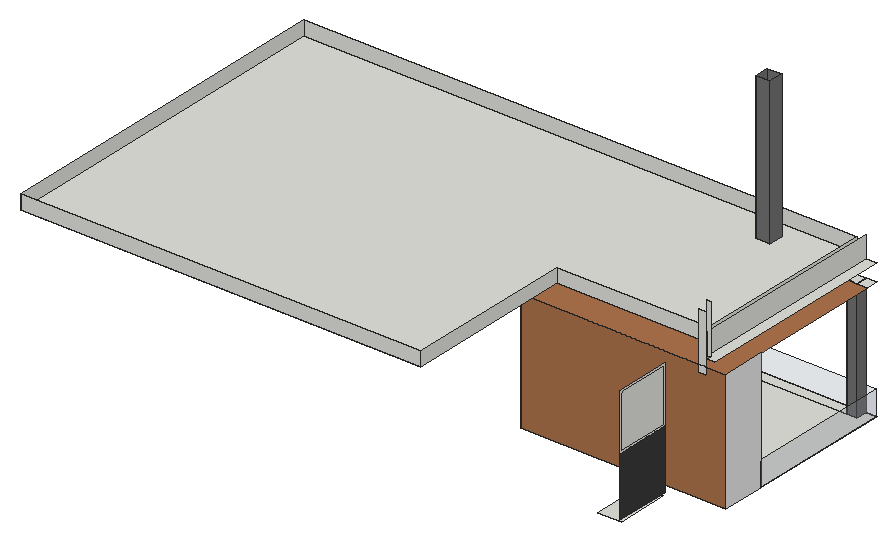
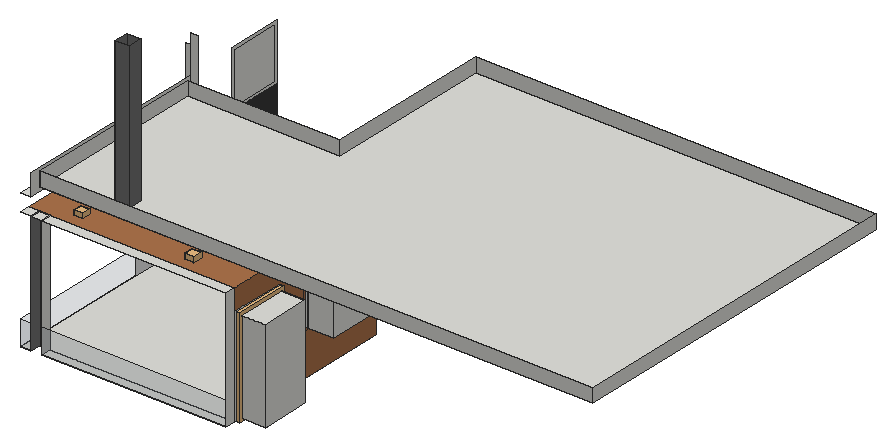
# SketchUp Ruby script. Lengths in inches.
U = 1.inch
M = Sketchup.active_model
def pt(a) = Geom::Point3d.new(a.map { |v| v * U })
def face(e, loops, mat)
  f = e.add_face(loops[0].map { |a| pt(a) })
  loops[1..].each { |l| e.add_face(l.map { |a| pt(a) }).erase! }
  f.material = f.back_material = mat if mat
  f
end
# faces: each face lists its corners as indices into pts; further lists are holes
def faces(e, pts, list, mat = nil) = list.each { |f| face(e, (f[0].is_a?(Array) ? f : [f]).map { |l| l.map { |i| pts[i] } }, mat) }
# xy, xz, yz: faces in a plane at the given z, y or x. An outline is a flat list of corners, or four numbers for a rectangle; further outlines are holes
def ring(l) = l.size == 4 ? [[l[0], l[1]], [l[2], l[1]], [l[2], l[3]], [l[0], l[3]]] : l.each_slice(2).to_a
def flat(e, list, mat, &to3) = list.each { |f| face(e, (f[0].is_a?(Array) ? f : [f]).map { |l| ring(l).map { |u, v| to3.(u, v) } }, mat) }
def xy(e, z, list, mat = nil) = flat(e, list, mat) { |x, y| [x, y, z] }
def xz(e, y, list, mat = nil) = flat(e, list, mat) { |x, z| [x, y, z] }
def yz(e, x, list, mat = nil) = flat(e, list, mat) { |y, z| [x, y, z] }
def lines(e, pts, list) = list.each { |a, b| e.add_line(pt(pts[a]), pt(pts[b])) }
# prism: a flat outline (further loops are holes) pulled along v
def prism(e, loops, v, mat = nil)
  f = face(e, loops, mat); d = Geom::Vector3d.new(v.map { |x| x * U })
  f.pushpull(f.normal.samedirection?(d) ? d.length : -d.length)
end
def box(e, o, s, mat = nil) = prism(e, [[o, [o[0] + s[0], o[1], o[2]], [o[0] + s[0], o[1] + s[1], o[2]], [o[0], o[1] + s[1], o[2]]]], [0, 0, s[2]], mat)
def at(x, y, z, deg = 0) = Geom::Transformation.translation(pt([x, y, z])) * Geom::Transformation.rotation(ORIGIN, Z_AXIS, deg.degrees)
def axes(o, x, y, z) = Geom::Transformation.new([*x, 0, *y, 0, *z, 0, *pt(o).to_a, 1])
def part(name) = M.definitions.add(name)
# library, detail: a bought-in or finely detailed component or shape, given as its bounding box
def library(name, o, s) = part(name).tap { |d| box(d.entities, o, s) }
def detail(e, o, s) = box(e.add_group.entities, o, s)
def put(e, d, t, mat = nil) = e.add_instance(d, t).tap { |i| i.material = mat if mat }
def group(e, t, mat = nil) = e.add_group.tap { |g| g.transformation = t; g.material = mat if mat }.entities
root = M.entities
M.materials.add("Batt_Blanket_Insulation_1K").color = [231, 231, 231]
M.materials.add("Glass_Basic_01").color = [161, 173, 186]
M.materials["Glass_Basic_01"].alpha = 0.25
M.materials.add("M05_Graphite_Haze").color = [114, 114, 114]
M.materials.add("ThomThom - Hat3").color = [58, 58, 58]
M.materials.add("Wood_Veneer_15_1K").color = [173, 116, 75]
c1 = library("porta+4",[0.2,-5.42,1.33],[46.55,4.72,83.21])
c2 = library("Group\#8",[0,0,0],[2.375,32.33,79.75])
c3 = library("Sphere Light\#4",[-4,-4,-4],[8,8,8])
c4 = library("Sphere Light\#6",[-4,-4,-4],[8,8,8])
c5 = library("Sphere Light\#5",[-3.88,-3.88,-3.88],[7.76,7.76,7.76])
c6 = library("Sphere Light\#3",[-3.6875,-3.6875,-3.6875],[7.375,7.375,7.375])
xy(root,135,[[312,153,486,153,486,312,477,312,477,303,312,303],[312,303,468,312]])
xy(root,138,[[288,258,312,300]])
xy(root,168.38,[[460.07,50,480,94]])
xy(root,174,[[288,186,312,228]])
xy(root,216,[[288,186,312,228],[288,258,312,300]])
xy(root,237,[[312,303,468,312],[468,303,477,312],[477,303,486,312]])
xy(root,237,[[[312,153,486,303],[452.97,284.875,454.01,284.98,454.99,285.36,455.83,285.97,456.49,286.78,456.91,287.73,457.08,288.76,456.97,289.8,456.6,290.78,455.99,291.625,455.17,292.28,454.22,292.71,453.19,292.87,452.15,292.76,451.18,292.39,450.33,291.78,449.67,290.97,449.25,290.01,449.08,288.98,449.19,287.94,449.5625,286.97,450.18,286.125,450.99,285.47,451.94,285.04],[452.97,190.99,454.01,191.1,454.99,191.47,455.83,192.09,456.49,192.9,456.91,193.85,457.08,194.88,456.97,195.92,456.6,196.9,455.99,197.74,455.17,198.4,454.22,198.83,453.19,198.99,452.15,198.88,451.18,198.51,450.33,197.9,449.67,197.09,449.25,196.13,449.08,195.1,449.19,194.0625,449.5625,193.09,450.18,192.24,450.99,191.58,451.94,191.16],[358.12,284.875,359.16,284.98,360.13,285.36,360.98,285.97,361.64,286.78,362.0625,287.73,362.23,288.76,362.12,289.8,361.75,290.78,361.13,291.625,360.32,292.28,359.37,292.71,358.34,292.87,357.3,292.76,356.32,292.39,355.48,291.78,354.82,290.97,354.4,290.01,354.23,288.98,354.34,287.94,354.71,286.97,355.32,286.125,356.14,285.47,357.09,285.04],[358.12,190.99,359.16,191.1,360.13,191.47,360.98,192.09,361.64,192.9,362.0625,193.85,362.23,194.88,362.12,195.92,361.75,196.9,361.13,197.74,360.32,198.4,359.37,198.83,358.34,198.99,357.3,198.88,356.32,198.51,355.48,197.9,354.82,197.09,354.4,196.13,354.23,195.1,354.34,194.0625,354.71,193.09,355.32,192.24,356.14,191.58,357.09,191.16]],[358.12,190.99,357.09,191.16,356.14,191.58,355.32,192.24,354.71,193.09,354.34,194.0625,354.23,195.1,354.4,196.13,354.82,197.09,355.48,197.9,356.32,198.51,357.3,198.88,358.34,198.99,359.37,198.83,360.32,198.4,361.13,197.74,361.75,196.9,362.12,195.92,362.23,194.88,362.0625,193.85,361.64,192.9,360.98,192.09,360.13,191.47,359.16,191.1],[452.97,190.99,451.94,191.16,450.99,191.58,450.18,192.24,449.5625,193.09,449.19,194.0625,449.08,195.1,449.25,196.13,449.67,197.09,450.33,197.9,451.18,198.51,452.15,198.88,453.19,198.99,454.22,198.83,455.17,198.4,455.99,197.74,456.6,196.9,456.97,195.92,457.08,194.88,456.91,193.85,456.49,192.9,455.83,192.09,454.99,191.47,454.01,191.1],[358.12,284.875,357.09,285.04,356.14,285.47,355.32,286.125,354.71,286.97,354.34,287.94,354.23,288.98,354.4,290.01,354.82,290.97,355.48,291.78,356.32,292.39,357.3,292.76,358.34,292.87,359.37,292.71,360.32,292.28,361.13,291.625,361.75,290.78,362.12,289.8,362.23,288.76,362.0625,287.73,361.64,286.78,360.98,285.97,360.13,285.36,359.16,284.98],[452.97,284.875,451.94,285.04,450.99,285.47,450.18,286.125,449.5625,286.97,449.19,287.94,449.08,288.98,449.25,290.01,449.67,290.97,450.33,291.78,451.18,292.39,452.15,292.76,453.19,292.87,454.22,292.71,455.17,292.28,455.99,291.625,456.6,290.78,456.97,289.8,457.08,288.76,456.91,287.73,456.49,286.78,455.83,285.97,454.99,285.36,454.01,284.98]],"Wood_Veneer_15_1K")
xy(root,252,[[480,141,486,141,486,312,477,312,477,144,480,144]])
xy(root,258,[[[6,6,345.33,6,345.33,150,474,150,474,306,6,306],[409.67,279.92,421.67,291.92]]])
xz(root,6,[[6,258,345.33,270]])
xz(root,132,[[480,246,486,252],[480,252,486,294]])
xz(root,144,[[477,252,480,294]])
xz(root,150,[[345.33,258,474,270]])
xz(root,153,[[312,135,486,237]],"Wood_Veneer_15_1K")
xz(root,186,[[288,174,312,216]])
xz(root,228,[[288,174,312,216]])
xz(root,258,[[288,138,312,216]])
xz(root,279.92,[[409.67,258,421.67,381]],"M05_Graphite_Haze")
xz(root,291.92,[[409.67,258,421.67,381]],"M05_Graphite_Haze")
xz(root,300,[[288,138,312,216]])
xz(root,303,[[468,135,477,237]],"M05_Graphite_Haze")
xz(root,306,[[6,258,474,270]])
xz(root,312,[[312,135,468,156],[477,135,486,156]],"Glass_Basic_01")
yz(root,6,[[6,258,306,270]])
yz(root,288,[[258,138,300,216],[186,174,228,216]])
yz(root,312,[[[255,135,303,219],[258,138,300,216]],[303,135,312,237]])
yz(root,312,[[[153,135,255,135,255,219,303,219,303,237,153,237],[183,171,231,219]],[[183,171,231,219],[186,174,228,216]]],"Wood_Veneer_15_1K")
yz(root,345.33,[[6,258,150,270]])
yz(root,409.67,[[279.92,258,291.92,381]],"M05_Graphite_Haze")
yz(root,421.67,[[279.92,258,291.92,381]],"M05_Graphite_Haze")
yz(root,468,[[303,135,312,237]])
yz(root,474,[[150,258,306,270]])
yz(root,477,[[144,252,312,270]])
yz(root,477,[[303,135,312,237]],"M05_Graphite_Haze")
yz(root,480,[[[48,220.76,96,268.76],[50,222.76,94,266.76]],[50,222.76,94,266.76]])
yz(root,480,[[48,170.38,96,220.76]],"ThomThom - Hat3")
yz(root,486,[[153,135,189.79,237]],"Batt_Blanket_Insulation_1K")
yz(root,486,[[189.79,135,312,156]],"Glass_Basic_01")
put(root,c1,at(307.72,254.8,133.66,90))
put(root,c2,axes([312,228,174],[-0.92105,0,0],[0,-1.29897,0],[0,0,0.52665]))
put(root,c3,at(358.23,288.875,237))
put(root,c4,at(453.08,194.99,237))
put(root,c5,at(357.94,194.98,237))
put(root,c6,at(452.64,288.9,237))
